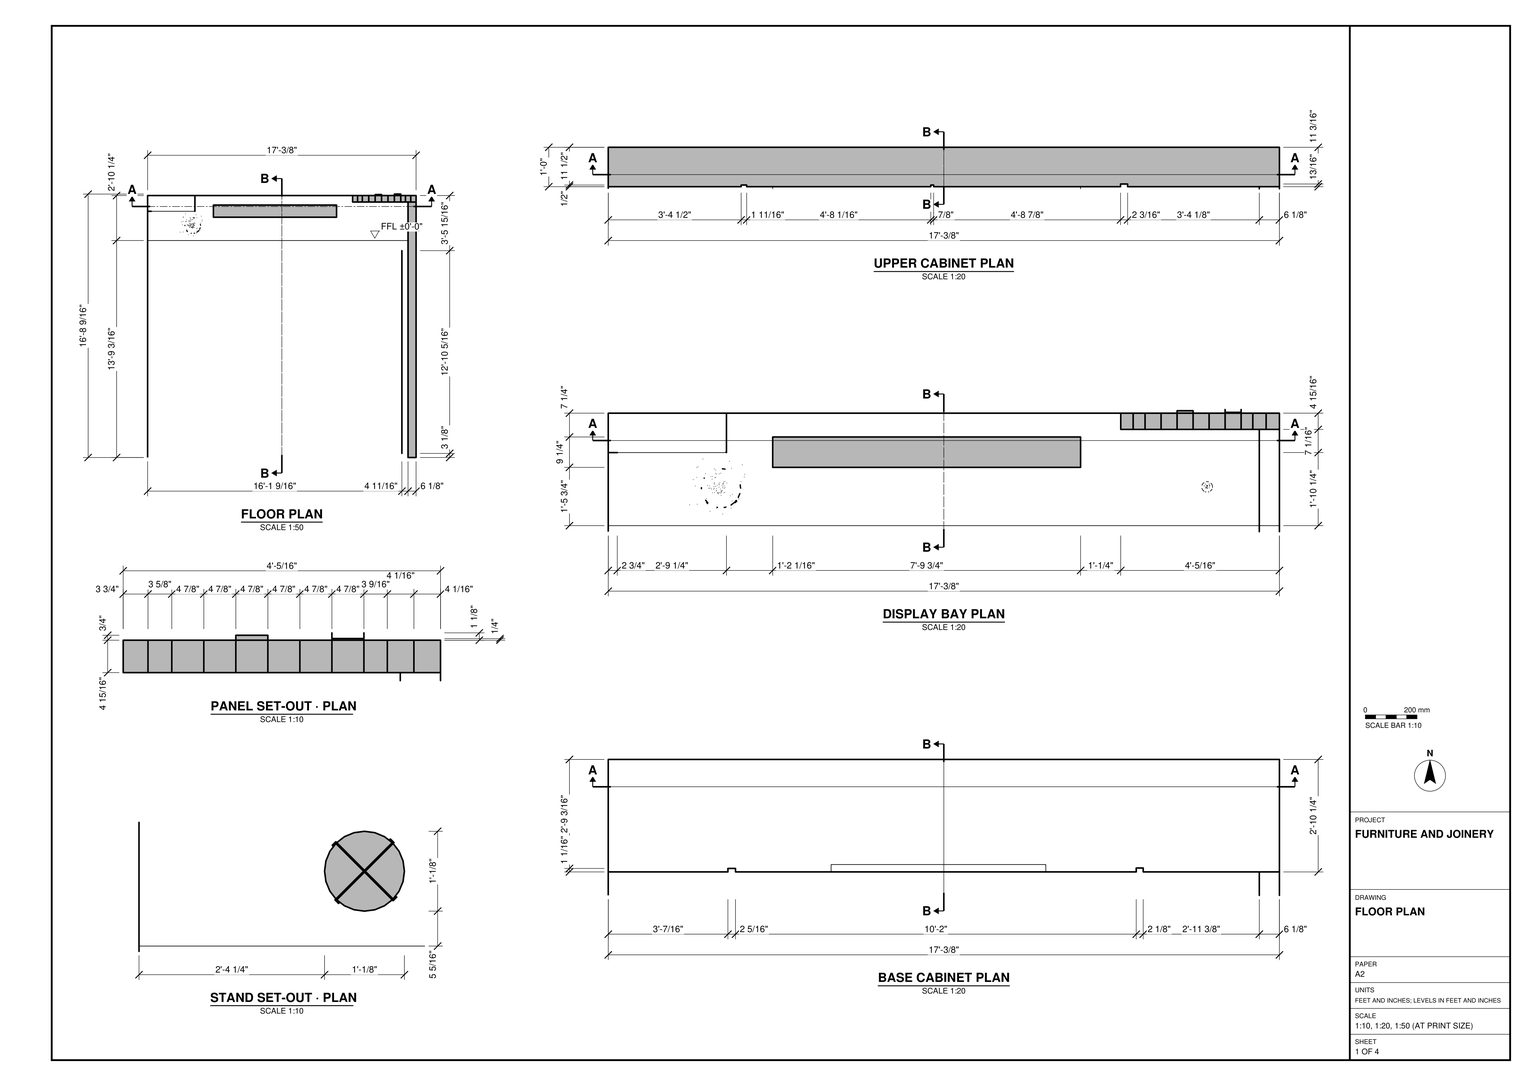
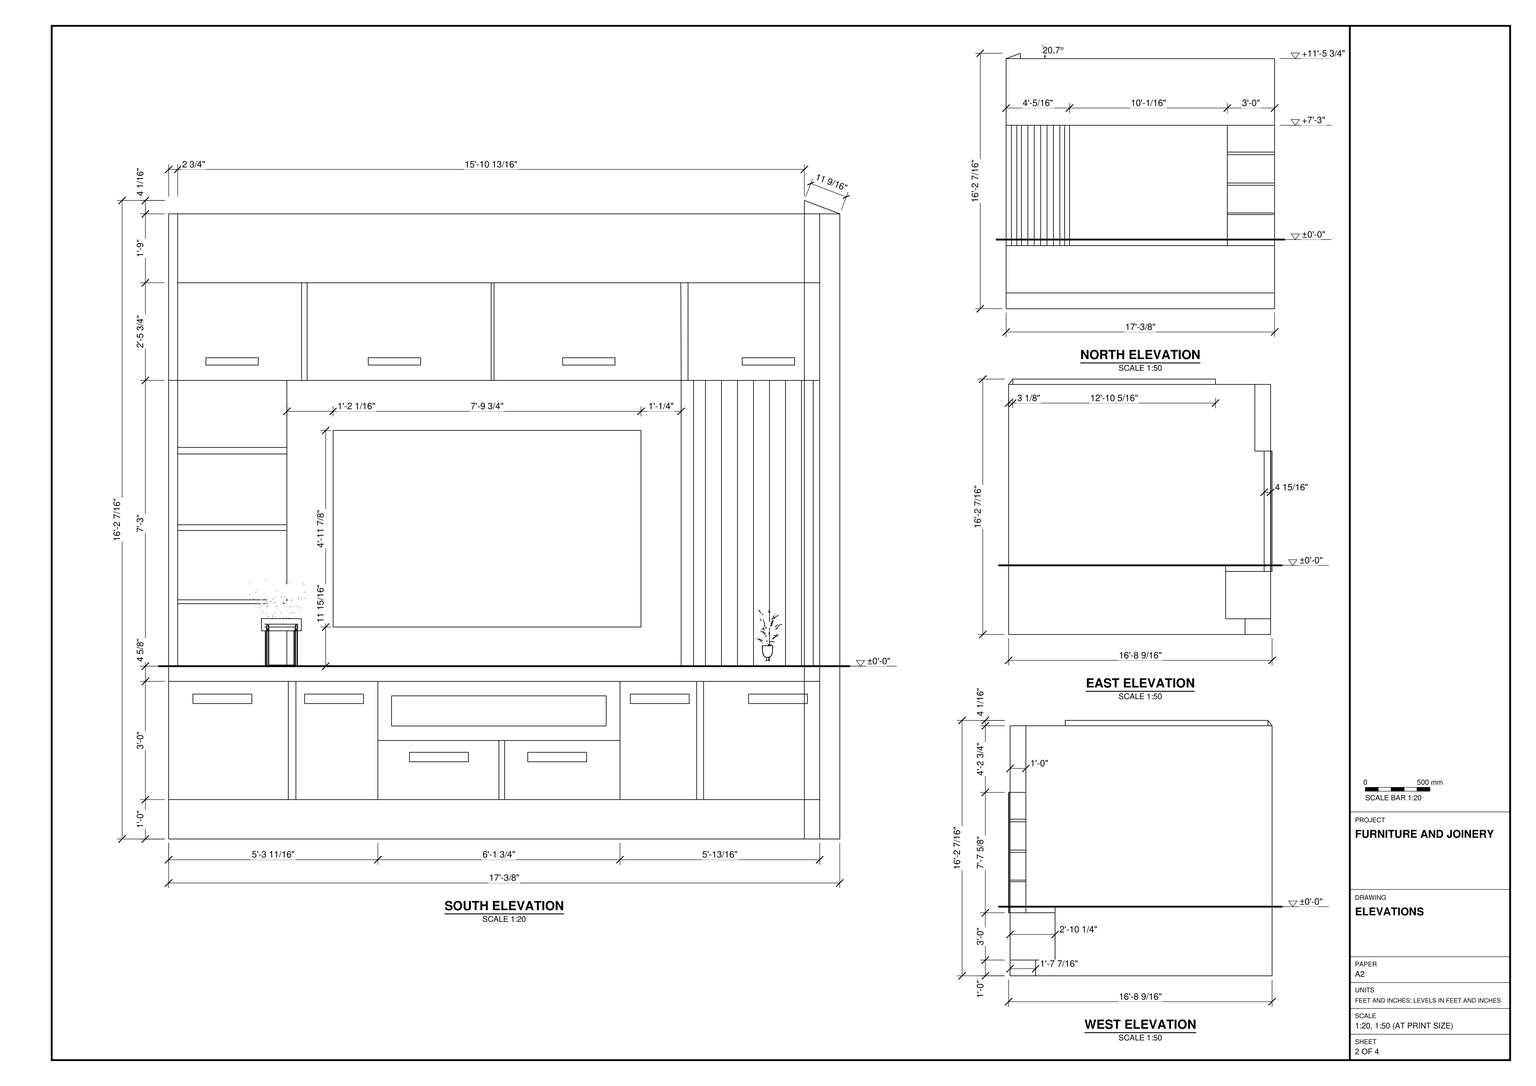
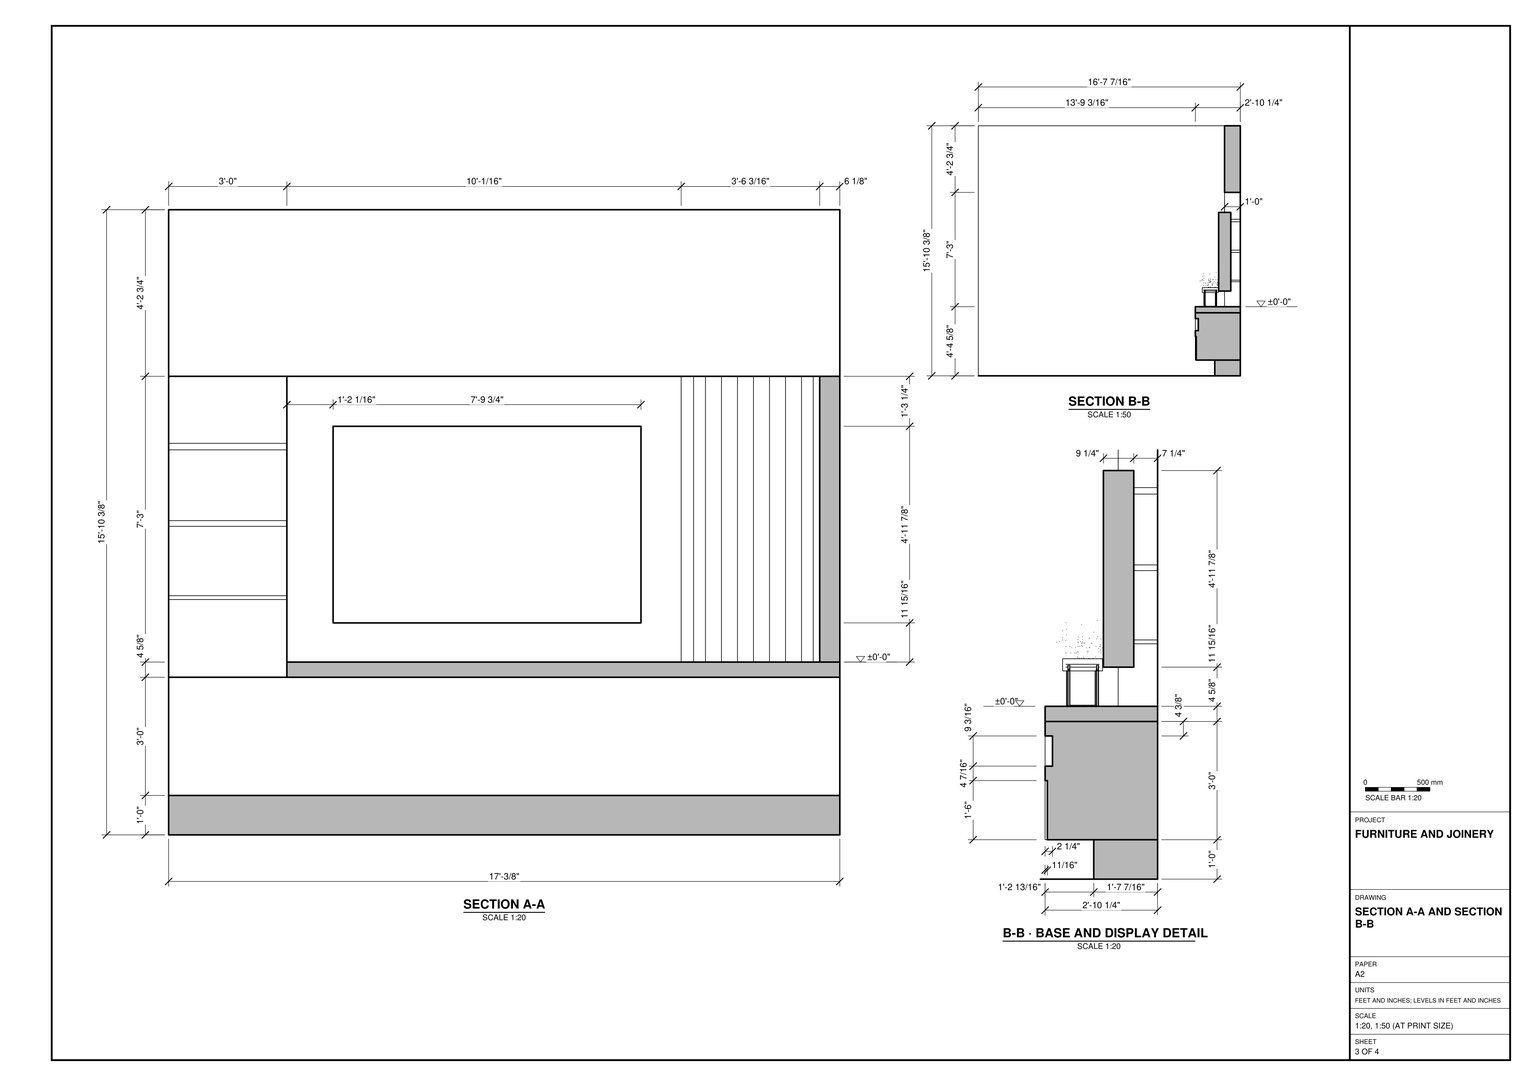
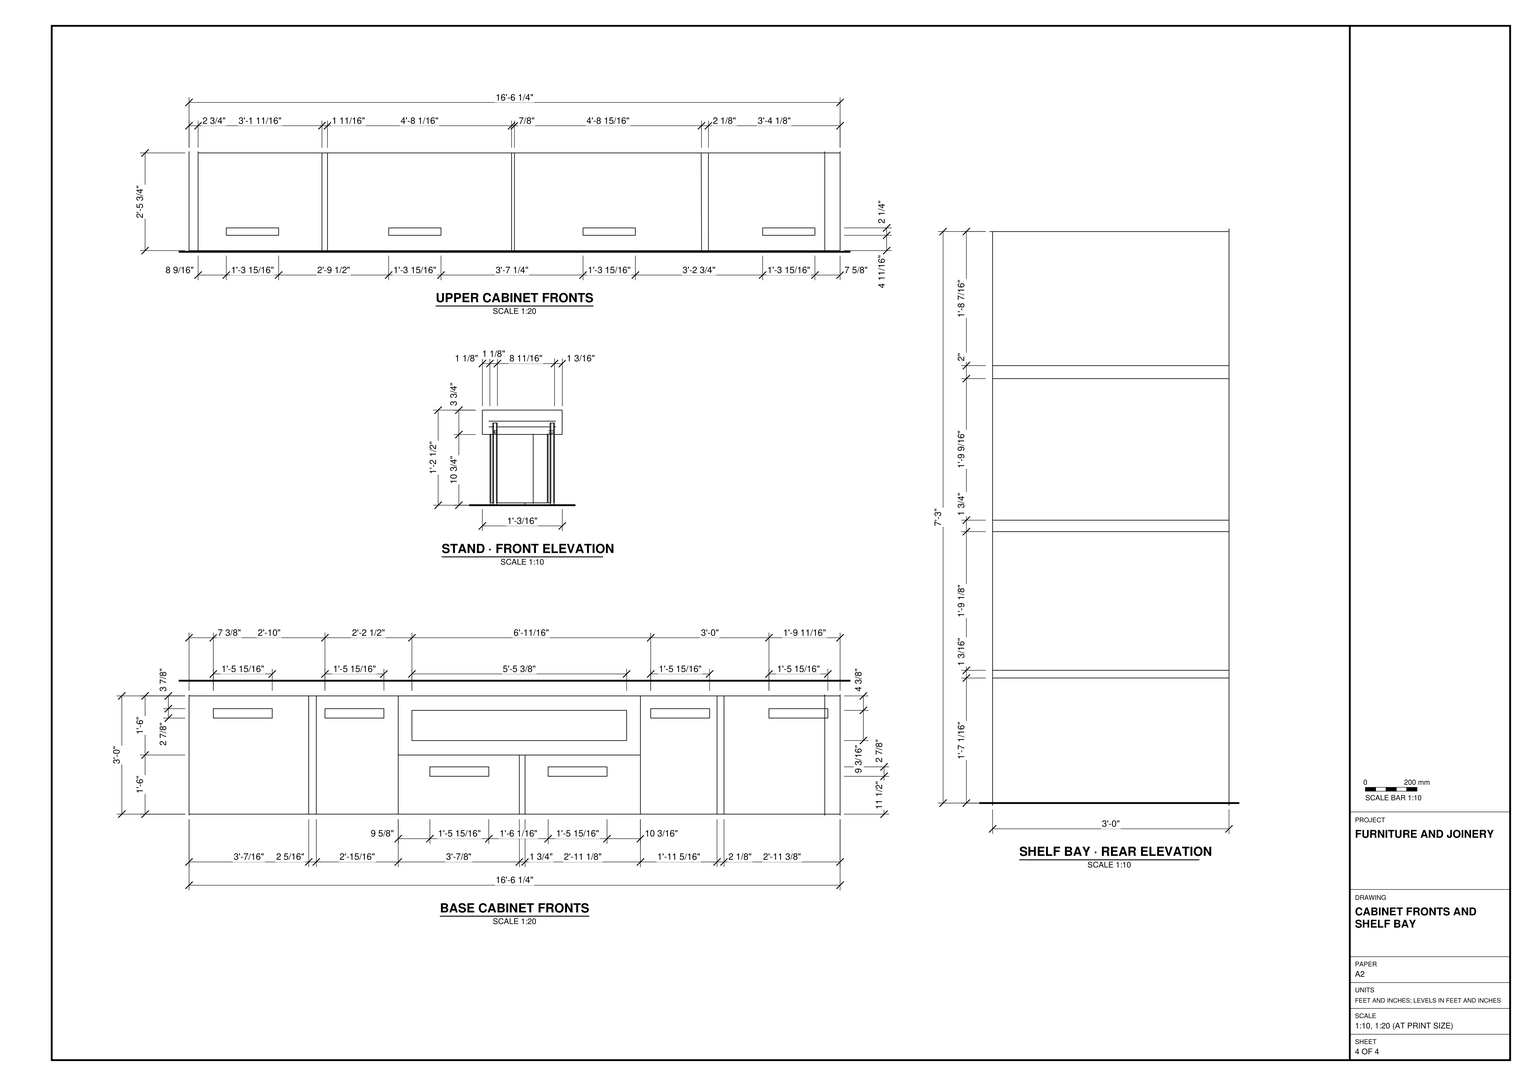
Build the fitted display wall in SketchUp from task_files/diagram_01.pdf. Work in feet and inches. The complete assembly, including the side return, measures 17'-3/8" across the cabinet fronts, 16'-8 9/16" from front to back and 16'-2 7/16" high. Use the marked level of ±0'-0" at the top of the base counter; the base cabinets and their plinth extend below this datum.

Use the south elevation to lay out the cabinet fronts and pulls. Form the recessed plinth, the full-width counter and the central base section with its broad horizontal inset above paired lower fronts. Between the counter and the upper cabinets, place open shelves on the left, a projecting rectangular display panel in the middle and narrow vertical panels on the right. Follow the panel set-out in plan for their widths and offsets. Include the band above the upper cabinet fronts. Use the plans and sections to distinguish the depths of the cabinets, shelves and display panel from the much longer right-hand return, keeping the return thickness as drawn.

Place the small stand and plants where shown; decor and loose items may be any suitable library components. Keep the surrounding elements and each joinery or furniture piece in separate groups or components, and use components for repeated parts. Save one SketchUp model as output_files/display_wall_with_base_and_upper_cabinets.skp.

# SketchUp Ruby script. Lengths in inches.
U = 1.inch
M = Sketchup.active_model
def pt(a) = Geom::Point3d.new(a.map { |v| v * U })
def face(e, loops, mat)
  f = e.add_face(loops[0].map { |a| pt(a) })
  loops[1..].each { |l| e.add_face(l.map { |a| pt(a) }).erase! }
  f.material = f.back_material = mat if mat
  f
end
# faces: each face lists its corners as indices into pts; further lists are holes
def faces(e, pts, list, mat = nil) = list.each { |f| face(e, (f[0].is_a?(Array) ? f : [f]).map { |l| l.map { |i| pts[i] } }, mat) }
# xy, xz, yz: faces in a plane at the given z, y or x. An outline is a flat list of corners, or four numbers for a rectangle; further outlines are holes
def ring(l) = l.size == 4 ? [[l[0], l[1]], [l[2], l[1]], [l[2], l[3]], [l[0], l[3]]] : l.each_slice(2).to_a
def flat(e, list, mat, &to3) = list.each { |f| face(e, (f[0].is_a?(Array) ? f : [f]).map { |l| ring(l).map { |u, v| to3.(u, v) } }, mat) }
def xy(e, z, list, mat = nil) = flat(e, list, mat) { |x, y| [x, y, z] }
def xz(e, y, list, mat = nil) = flat(e, list, mat) { |x, z| [x, y, z] }
def yz(e, x, list, mat = nil) = flat(e, list, mat) { |y, z| [x, y, z] }
def lines(e, pts, list) = list.each { |a, b| e.add_line(pt(pts[a]), pt(pts[b])) }
# prism: a flat outline (further loops are holes) pulled along v
def prism(e, loops, v, mat = nil)
  f = face(e, loops, mat); d = Geom::Vector3d.new(v.map { |x| x * U })
  f.pushpull(f.normal.samedirection?(d) ? d.length : -d.length)
end
def box(e, o, s, mat = nil) = prism(e, [[o, [o[0] + s[0], o[1], o[2]], [o[0] + s[0], o[1] + s[1], o[2]], [o[0], o[1] + s[1], o[2]]]], [0, 0, s[2]], mat)
def at(x, y, z, deg = 0) = Geom::Transformation.translation(pt([x, y, z])) * Geom::Transformation.rotation(ORIGIN, Z_AXIS, deg.degrees)
def axes(o, x, y, z) = Geom::Transformation.new([*x, 0, *y, 0, *z, 0, *pt(o).to_a, 1])
def part(name) = M.definitions.add(name)
# library, detail: a bought-in or finely detailed component or shape, given as its bounding box
def library(name, o, s) = part(name).tap { |d| box(d.entities, o, s) }
def detail(e, o, s) = box(e.add_group.entities, o, s)
def put(e, d, t, mat = nil) = e.add_instance(d, t).tap { |i| i.material = mat if mat }
def group(e, t, mat = nil) = e.add_group.tap { |g| g.transformation = t; g.material = mat if mat }.entities
root = M.entities
M.materials.add("CORTINA").color = [173, 164, 148]
M.materials.add("[Color A01]").color = [255, 204, 204]
M.materials.add("[Color M00]").color = [255, 255, 255]
M.materials.add("[Color M01]").color = [226, 226, 226]
M.materials.add("[Color M08]").color = [30, 30, 30]
M.materials.add("[Fencing Wood Old]").color = [132, 128, 126]
M.materials.add("[Formica Laminate Dark]").color = [50, 53, 60]
M.materials.add("[Formica Speckled Grey]").color = [94, 105, 111]
M.materials.add("[Marble Carrara Gold Floor Tile]").color = [225, 223, 217]
M.materials.add("[Textile_Leaves_Green]").color = [49, 73, 8]
M.materials.add("[Vegetation Bark Ponderosa]").color = [158, 116, 100]
M.materials.add("[Wood Bamboo]").color = [177, 105, 43]
M.materials.add("[Wood Board Cork]").color = [215, 201, 115]
M.materials.add("[Wood Fence]").color = [20, 19, 18]
M.materials.add("[Wood Floor Light]").color = [204, 176, 127]
M.materials.add("[Wood Floor Parquet]").color = [145, 89, 39]
M.materials.add("[Wood Plywood Knots]").color = [137, 122, 41]
c1 = library("Decorative Plant",[-0.35,-0.24,0],[4.14,4.48,6.875])
c2 = part("Cortina")
xz(c2.entities,0,[[0,0,157.48,157.48]],"CORTINA")
c3 = part("curtain")
put(c3.entities,c2,at(0,0,0))
c4 = part("cof")
g1 = group(c4.entities,at(3.92,3.93,-15.01))
xy(g1,0,[[1.97,-0.53,12.72,10.22,22.38,0.56,23.8,1.97,13.05,12.72,22.72,22.38,21.3,23.8,10.55,13.05,0.89,22.72,-0.53,21.3,10.22,10.55,0.56,0.89]],"[Wood Fence]")
xy(g1,0.47,[[1.99,-0.5,0.58,0.91,10.22,10.55,-0.5,21.28,0.91,22.69,10.55,13.05,21.28,23.78,22.69,22.36,13.05,12.72,23.78,1.99,22.36,0.58,12.72,10.22]],"[Wood Fence]")
xy(g1,14.49,[[0.67,0.33,11.64,11.3,22.61,0.33,22.9375,0.67,11.97,11.64,22.9375,22.61,22.61,22.9375,11.64,11.97,0.67,22.9375,0.33,22.61,11.3,11.64,0.33,0.67]],"[Wood Fence]")
xy(g1,14.96,[[0.67,0.33,0.33,0.67,11.3,11.64,0.33,22.61,0.67,22.93,11.64,11.97,22.61,22.9375,22.77,22.77,22.9375,22.61,11.97,11.64,22.93,0.67,22.77,0.5,22.6,0.34,11.64,11.3],[22.6,0.34,22.93,0.67,22.77,0.5],[22.77,0.5,22.93,0.67,24.02,1.75]],"[Wood Fence]")
xy(g1,16.54,[[1.42,-1.08,0,0.33,0.33,0.67,1.75,-0.75],[22.9375,0,22.61,0.33,22.77,0.5,24.02,1.75,24.36,1.42],[-0.75,21.52,-1.08,21.86,0.33,23.27,0.67,22.9375,0.5,22.77],[22.9375,22.61,22.77,22.77,21.52,24.02,21.86,24.36,23.27,22.9375]],"[Wood Fence]")
p = [[12.72,10.22,0],[1.97,-0.53,0],[1.83,-0.67,0.03],[1.69,-0.8,0.11],[1.58,-0.92,0.23],[1.49,-1.01,0.39],
  [1.44,-1.0625,0.58],[1.42,-1.08,0.79],[1.42,-1.08,16.54],[1.75,-0.75,16.54],[1.75,-0.75,14.96],[1.75,-0.75,14.49],
  [1.75,-0.75,0.82],[1.76,-0.74,0.71],[1.78,-0.72,0.63],[1.82,-0.68,0.57],[1.86,-0.64,0.52],[1.92,-0.58,0.49],
  [1.99,-0.5,0.47],[12.72,10.22,0.47],[0.28,0.61,0.11],[0.41,0.75,0.03],[0.56,0.89,0],[22.36,0.58,0.47],
  [22.4375,0.5,0.49],[22.49,0.45,0.52],[22.54,0.4,0.57],[22.57,0.37,0.63],[22.59,0.34,0.71],[22.61,0.33,0.82],
  [22.61,0.33,14.49],[22.6,0.34,14.96],[22.61,0.33,16.54],[22.9375,0,16.54],[22.9375,0,0.79],[22.92,0.02,0.58],
  [22.86,0.07,0.39],[22.78,0.16,0.23],[22.66,0.28,0.11],[22.53,0.41,0.03],[22.38,0.56,0],[10.22,10.55,0.47],
  [0.58,0.91,0.47],[0.5,0.83,0.49],[0.45,0.78,0.52],[0.4,0.74,0.57],[0.37,0.7,0.63],[0.34,0.68,0.71],
  [0.33,0.67,0.82],[0.33,0.67,14.49],[0.33,0.67,14.96],[0.33,0.67,16.54],[0,0.33,16.54],[0,0.33,0.79],
  [0.02,0.35,0.58],[0.07,0.41,0.39],[0.16,0.5,0.23],[10.22,10.55,0],[24.08,1.69,0.11],[23.94,1.83,0.03],
  [23.8,1.97,0],[13.05,12.72,0],[24.19,1.58,0.23],[24.28,1.49,0.39],[24.34,1.44,0.58],[24.36,1.42,0.79],
  [24.36,1.42,16.54],[24.02,1.75,16.54],[24.02,1.75,14.96],[24.02,1.75,14.49],[24.02,1.75,0.82],[24.01,1.76,0.71],
  [23.99,1.78,0.63],[23.95,1.82,0.57],[23.91,1.86,0.52],[23.86,1.92,0.49],[23.78,1.99,0.47],[13.05,12.72,0.47],
  [-0.53,21.3,0],[-0.67,21.44,0.03],[-0.8,21.58,0.11],[-0.92,21.69,0.23],[-1.01,21.78,0.39],[-1.0625,21.84,0.58],
  [-1.08,21.86,0.79],[-1.08,21.86,16.54],[-0.75,21.52,16.54],[-0.75,21.52,14.96],[-0.75,21.52,14.49],[-0.75,21.52,0.82],
  [-0.74,21.51,0.71],[-0.72,21.49,0.63],[-0.68,21.46,0.57],[-0.64,21.41,0.52],[-0.58,21.36,0.49],[-0.5,21.28,0.47],
  [22.69,22.36,0.47],[22.77,22.4375,0.49],[22.83,22.49,0.52],[22.87,22.54,0.57],[22.91,22.57,0.63],[22.93,22.59,0.71],
  [22.9375,22.61,0.82],[22.9375,22.61,14.49],[22.9375,22.61,14.96],[22.9375,22.61,16.54],[23.27,22.9375,16.54],[23.27,22.9375,0.79],
  [23.25,22.92,0.58],[23.2,22.86,0.39],[23.11,22.78,0.23],[22.99,22.66,0.11],[22.86,22.53,0.03],[22.72,22.38,0],
  [10.55,13.05,0.47],[0.91,22.69,0.47],[0.83,22.77,0.49],[0.78,22.83,0.52],[0.74,22.87,0.57],[0.7,22.91,0.63],
  [0.68,22.93,0.71],[0.67,22.9375,0.82],[0.67,22.9375,14.49],[0.67,22.93,14.96],[0.67,22.9375,16.54],[0.33,23.27,16.54],
  [0.33,23.27,0.79],[0.35,23.25,0.58],[0.41,23.2,0.39],[0.5,23.11,0.23],[0.61,22.99,0.11],[0.75,22.86,0.03],
  [0.89,22.72,0],[10.55,13.05,0],[21.3,23.8,0],[21.44,23.94,0.03],[21.58,24.08,0.11],[21.69,24.19,0.23],
  [21.78,24.28,0.39],[21.84,24.34,0.58],[21.86,24.36,0.79],[21.86,24.36,16.54],[21.52,24.02,16.54],[21.52,24.02,14.96],
  [21.52,24.02,14.49],[21.52,24.02,0.82],[21.51,24.01,0.71],[21.49,23.99,0.63],[21.46,23.95,0.57],[21.41,23.91,0.52],
  [21.36,23.86,0.49],[21.28,23.78,0.47],[0.67,0.33,14.49],[22.9375,0.67,14.49],[0.33,22.61,14.49],[22.61,22.9375,14.49],
  [0.67,0.33,14.96],[0.5,0.5,14.96],[11.64,11.3,14.49],[11.64,11.3,14.96],[22.93,0.67,14.96],[11.3,11.64,14.96],
  [11.3,11.64,14.49],[11.97,11.64,14.49],[11.97,11.64,14.96],[0.33,22.61,14.96],[11.64,11.97,14.96],[11.64,11.97,14.49],
  [22.61,22.9375,14.96],[22.77,22.77,14.96],[0.5,0.5,16.54],[22.77,0.5,14.96],[22.77,0.5,16.54],[0.5,22.77,16.54],
  [0.5,22.77,14.96],[22.77,22.77,16.54]]
faces(g1,p,[[0,1,2,3,4,5,6,7,8,9,10,11,12,13,14,15,16,17,18,19],[20,3,2,21],[21,2,1,22],[19,23,24,25,26,27,28,29,30,31,32,33,34,35,36,37,38,39,40,0],[41,42,43,44,45,46,47,48,49,50,51,52,53,54,55,56,20,21,22,57],[39,38,58,59],[40,39,59,60],[61,60,59,58,62,63,64,65,66,67,68,69,70,71,72,73,74,75,76,77],
  [57,78,79,80,81,82,83,84,85,86,87,88,89,90,91,92,93,94,95,41],[77,96,97,98,99,100,101,102,103,104,105,106,107,108,109,110,111,112,113,61],[114,115,116,117,118,119,120,121,122,123,124,125,126,127,128,129,130,131,132,133],[133,134,135,136,137,138,139,140,141,142,143,144,145,146,147,148,149,150,151,114],[131,79,78,132],[130,80,79,131],[113,112,135,134],[112,111,136,135],
  [56,4,3,20],[38,37,62,58],[129,81,80,130],[111,110,137,136],[55,5,4,56],[37,36,63,62],[128,82,81,129],[110,109,138,137],
  [54,6,5,55],[36,35,64,63],[127,83,82,128],[109,108,139,138],[44,16,15,45],[43,17,16,44],[42,18,17,43],[25,24,75,74],
  [26,25,74,73],[24,23,76,75],[115,95,94,116],[117,93,92,118],[116,94,93,117],[97,96,151,150],[98,97,150,149],[99,98,149,148],
  [53,7,6,54],[46,14,13,47],[45,15,14,46],[35,34,65,64],[28,27,72,71],[27,26,73,72],[119,91,90,120],[118,92,91,119],
  [126,84,83,127],[100,99,148,147],[101,100,147,146],[108,107,140,139],[47,13,12,48],[29,28,71,70],[120,90,89,121],[102,101,146,145],
  [52,8,7,53],[49,48,12,11,152],[34,33,66,65],[30,29,70,69,153],[122,121,89,88,154],[125,85,84,126],[103,102,145,144,155],[107,106,141,140],
  [156,152,11,10],[156,152,49,50,157],[158,152,156,159],[159,31,30,158],[30,31,153],[160,153,31],[161,50,49,162],[163,153,160,164],
  [153,69,160],[68,160,69],[162,154,165,161],[164,104,103,163],[166,123,122,167],[167,155,168,166],[165,154,88,87],[122,123,154],
  [165,154,123],[103,104,169,168,155],[168,155,144,143],[9,170,157,156,10],[171,172,31],[32,31,172],[50,157,170,51],[172,171,68],
  [67,172,68],[86,173,174,165,87],[104,169,175,105],[174,173,123],[124,123,173],[142,175,169,168,143]],"[Wood Fence]")
c5 = part("Component")
g2 = group(c5.entities,at(0,0,0),"[Vegetation Bark Ponderosa]")
put(g2,c4,axes([-4.91,2.93,5.08],[0.07854,0,0],[0,0.07854,0],[0,0,0.34302]),"[Fencing Wood Old]")
g3 = group(g2,at(-4.92,2.91,4.8125),"[Vegetation Bark Ponderosa]")
xy(g3,0.52,[[1.24,0.04,1.55,0.08,1.83,0.2,2.08,0.39,2.27,0.64,2.39,0.93,2.43,1.24,2.39,1.55,2.27,1.83,2.08,2.08,1.83,2.27,1.55,2.39,1.24,2.43,0.93,2.39,0.64,2.27,0.39,2.08,0.2,1.83,0.08,1.55,0.04,1.24,0.08,0.93,0.2,0.64,0.39,0.39,0.64,0.2,0.93,0.08]],"[Vegetation Bark Ponderosa]")
xy(g3,0.92,[[1.24,0.04,1.55,0.08,1.83,0.2,2.08,0.39,2.27,0.64,2.39,0.93,2.43,1.24,2.39,1.55,2.27,1.83,2.08,2.08,1.83,2.27,1.55,2.39,1.24,2.43,0.93,2.39,0.64,2.27,0.39,2.08,0.2,1.83,0.08,1.55,0.04,1.24,0.08,0.93,0.2,0.64,0.39,0.39,0.64,0.2,0.93,0.08]],"[Vegetation Bark Ponderosa]")
xy(g3,1.68,[[[1.24,0,1.56,0.04,1.86,0.17,2.11,0.36,2.31,0.62,2.43,0.92,2.47,1.24,2.43,1.56,2.31,1.86,2.11,2.11,1.86,2.31,1.56,2.43,1.24,2.47,0.92,2.43,0.62,2.31,0.36,2.11,0.17,1.86,0.04,1.56,0,1.24,0.04,0.92,0.17,0.62,0.36,0.36,0.62,0.17,0.92,0.04],[1.24,0.04,0.93,0.08,0.64,0.2,0.39,0.39,0.2,0.64,0.08,0.93,0.04,1.24,0.08,1.55,0.2,1.83,0.39,2.08,0.64,2.27,0.93,2.39,1.24,2.43,1.55,2.39,1.83,2.27,2.08,2.08,2.27,1.83,2.39,1.55,2.43,1.24,2.39,0.93,2.27,0.64,2.08,0.39,1.83,0.2,1.55,0.08]]],"[Color M00]")
p = [[0.62,0.17,0],[0.92,0.04,0],[0.92,0.04,1.68],[0.62,0.17,1.68],[1.24,0,0],[1.24,0,1.68],
  [1.56,0.04,0],[1.56,0.04,1.68],[1.86,0.17,0],[1.86,0.17,1.68],[0.36,0.36,0],[0.36,0.36,1.68],
  [2.11,0.36,0],[2.11,0.36,1.68],[0.17,0.62,0],[0.17,0.62,1.68],[2.31,0.62,0],[2.31,0.62,1.68],
  [0.04,0.92,0],[0.04,0.92,1.68],[2.43,0.92,0],[2.43,0.92,1.68],[0,1.24,0],[0,1.24,1.68],
  [2.47,1.24,0],[2.47,1.24,1.68],[0.04,1.56,0],[0.04,1.56,1.68],[2.43,1.56,0],[2.43,1.56,1.68],
  [0.17,1.86,0],[0.17,1.86,1.68],[2.31,1.86,0],[2.31,1.86,1.68],[0.36,2.11,0],[0.36,2.11,1.68],
  [2.11,2.11,0],[2.11,2.11,1.68],[0.62,2.31,0],[0.62,2.31,1.68],[1.86,2.31,0],[1.86,2.31,1.68],
  [0.92,2.43,0],[0.92,2.43,1.68],[1.56,2.43,0],[1.56,2.43,1.68],[1.24,2.47,0],[1.24,2.47,1.68],
  [1.24,0.04,0.52],[0.93,0.08,0.52],[0.93,0.08,0.92],[1.24,0.04,0.92],[1.55,0.08,0.52],[1.55,0.08,0.92],
  [0.64,0.2,0.52],[0.64,0.2,0.92],[1.83,0.2,0.52],[1.83,0.2,0.92],[0.39,0.39,0.52],[0.39,0.39,0.92],
  [2.08,0.39,0.52],[2.08,0.39,0.92],[0.2,0.64,0.52],[0.2,0.64,0.92],[2.27,0.64,0.52],[2.27,0.64,0.92],
  [0.08,0.93,0.52],[0.08,0.93,0.92],[2.39,0.93,0.52],[2.39,0.93,0.92],[0.04,1.24,0.52],[0.04,1.24,0.92],
  [2.43,1.24,0.52],[2.43,1.24,0.92],[0.08,1.55,0.52],[0.08,1.55,0.92],[2.39,1.55,0.52],[2.39,1.55,0.92],
  [0.2,1.83,0.52],[0.2,1.83,0.92],[2.27,1.83,0.52],[2.27,1.83,0.92],[0.39,2.08,0.52],[0.39,2.08,0.92],
  [2.08,2.08,0.52],[2.08,2.08,0.92],[0.64,2.27,0.52],[0.64,2.27,0.92],[1.83,2.27,0.52],[1.83,2.27,0.92],
  [0.93,2.39,0.52],[0.93,2.39,0.92],[1.55,2.39,0.52],[1.55,2.39,0.92],[1.24,2.43,0.52],[1.24,2.43,0.92],
  [1.24,0.04,1.68],[0.93,0.08,1.68],[1.55,0.08,1.68],[0.64,0.2,1.68],[1.83,0.2,1.68],[0.39,0.39,1.68],
  [2.08,0.39,1.68],[0.2,0.64,1.68],[2.27,0.64,1.68],[0.08,0.93,1.68],[2.39,0.93,1.68],[0.04,1.24,1.68],
  [2.43,1.24,1.68],[0.08,1.55,1.68],[2.39,1.55,1.68],[0.2,1.83,1.68],[2.27,1.83,1.68],[0.39,2.08,1.68],
  [2.08,2.08,1.68],[0.64,2.27,1.68],[1.83,2.27,1.68],[0.93,2.39,1.68],[1.55,2.39,1.68],[1.24,2.43,1.68]]
faces(g3,p,[[0,1,2,3],[1,4,5,2],[4,6,7,5],[6,8,9,7],[10,0,3,11],[8,12,13,9],[14,10,11,15],[12,16,17,13],
  [18,14,15,19],[16,20,21,17],[22,18,19,23],[20,24,25,21],[26,22,23,27],[24,28,29,25],[30,26,27,31],[28,32,33,29],
  [34,30,31,35],[32,36,37,33],[38,34,35,39],[36,40,41,37],[42,38,39,43],[40,44,45,41],[46,42,43,47],[44,46,47,45],
  [96,51,50,97],[98,53,51,96],[97,50,55,99],[100,57,53,98],[99,55,59,101],[102,61,57,100],[101,59,63,103],[104,65,61,102],
  [103,63,67,105],[106,69,65,104],[105,67,71,107],[108,73,69,106],[107,71,75,109],[110,77,73,108],[109,75,79,111],[112,81,77,110],
  [111,79,83,113],[114,85,81,112],[113,83,87,115],[116,89,85,114],[115,87,91,117],[118,93,89,116],[117,91,95,119],[119,95,93,118]],"[Color M00]")
faces(g3,p,[[48,49,50,51],[52,48,51,53],[49,54,55,50],[56,52,53,57],[54,58,59,55],[60,56,57,61],[58,62,63,59],[64,60,61,65],
  [62,66,67,63],[68,64,65,69],[66,70,71,67],[72,68,69,73],[70,74,75,71],[76,72,73,77],[74,78,79,75],[80,76,77,81],
  [78,82,83,79],[84,80,81,85],[82,86,87,83],[88,84,85,89],[86,90,91,87],[92,88,89,93],[90,94,95,91],[94,92,93,95]],"[Vegetation Bark Ponderosa]")
c6 = part("Plant leaf")
p = [[4.001,2.211,9.034],[3.964,2.195,9.038],[2.645,1.619,9.164],[2.684,1.471,8.407],[2.728,1.324,7.649],[2.778,1.18,6.891],
  [2.834,1.039,6.133],[2.895,0.9,5.374],[2.962,0.764,4.614],[3.035,0.631,3.855],[3.114,0.499,3.095],[3.198,0.371,2.334],
  [3.288,0.245,1.574],[3.383,0.121,0.8125],[3.485,0,0.051],[3.964,0.209,0.004],[4.001,0.225,0],[3.926,2.211,9.034],
  [3.926,0.225,0],[4.443,0,0.051],[4.544,0.121,0.8125],[4.64,0.245,1.574],[4.73,0.371,2.334],[4.814,0.499,3.095],
  [4.892,0.631,3.855],[4.965,0.764,4.614],[5.032,0.9,5.374],[5.094,1.039,6.133],[5.15,1.18,6.891],[5.2,1.324,7.649],
  [5.244,1.471,8.407],[5.283,1.619,9.164],[4.001,5.314,17.748],[3.964,5.299,17.754],[2.264,4.583,18.009],[2.638,1.639,9.243],
  [3.964,2.196,9.04],[2.638,1.638,9.241],[5.29,1.639,9.243],[5.29,1.638,9.241],[3.926,5.314,17.748],[5.664,4.583,18.009],
  [4.001,9.442,26.026],[3.964,9.427,26.034],[2.001,8.641,26.425],[1.959,8.281,25.744],[1.929,7.925,25.061],[1.91,7.574,24.375],
  [1.903,7.227,23.686],[1.907,6.884,22.996],[1.922,6.547,22.303],[1.949,6.213,21.608],[1.987,5.885,20.911],[2.036,5.561,20.211],
  [2.097,5.242,19.51],[2.17,4.928,18.807],[2.253,4.618,18.102],[3.964,5.299,17.756],[5.674,4.618,18.102],[3.926,9.442,26.026],
  [5.758,4.928,18.807],[5.83,5.242,19.51],[5.891,5.561,20.211],[5.941,5.885,20.911],[5.979,6.213,21.608],[6.006,6.547,22.303],
  [6.021,6.884,22.996],[6.025,7.227,23.686],[6.018,7.574,24.375],[5.999,7.925,25.061],[5.969,8.281,25.744],[5.927,8.641,26.425],
  [3.964,9.428,26.035],[2.001,8.688,26.507],[5.927,8.688,26.507],[4.001,14.357,33.862],[3.964,14.343,33.871],[2.87,13.929,34.131],
  [2.735,13.47,33.513],[2.611,13.015,32.891],[2.499,12.564,32.267],[2.398,12.117,31.639],[2.309,11.674,31.008],[2.23,11.235,30.374],
  [2.164,10.8,29.737],[2.108,10.369,29.097],[2.064,9.942,28.454],[2.032,9.52,27.808],[2.011,9.102,27.159],[3.926,14.357,33.862],
  [5.917,9.102,27.159],[5.896,9.52,27.808],[5.863,9.942,28.454],[5.819,10.369,29.097],[5.764,10.8,29.737],[5.697,11.235,30.374],
  [5.619,11.674,31.008],[5.53,12.117,31.639],[5.429,12.564,32.267],[5.316,13.015,32.891],[5.193,13.47,33.513],[5.058,13.929,34.131],
  [3.964,14.344,33.873],[2.869,13.975,34.194],[5.058,13.975,34.194],[4.001,20.377,40.886],[3.97,19.863,40.308],[3.964,19.793,40.23],
  [3.927,19.346,39.734],[3.872,18.825,39.163],[3.806,18.3,38.596],[3.729,17.771,38.033],[3.64,17.24,37.473],[3.54,16.704,36.917],
  [3.428,16.165,36.365],[3.306,15.623,35.817],[3.171,15.077,35.272],[3.026,14.528,34.731],[3.926,20.377,40.886],[4.902,14.528,34.731],
  [4.756,15.077,35.272],[4.622,15.623,35.817],[4.499,16.165,36.365],[4.388,16.704,36.917],[4.288,17.24,37.473],[4.199,17.771,38.033],
  [4.122,18.3,38.596],[4.056,18.825,39.163],[4.001,19.346,39.734],[3.958,19.863,40.308]]
faces(c6.entities,p,[[0,1,2,3,4,5,6,7,8,9,10,11,12,13,14,15,16],[1,17,18,15,19,20,21,22,23,24,25,26,27,28,29,30,31],[32,33,34,35,36,0],[36,35,37,2,1,0],[38,36,17,1,31,39],[33,40,17,36,38,41],[42,43,44,45,46,47,48,49,50,51,52,53,54,55,56,57,32],[57,56,34,33,32],
  [58,57,40,33,41],[43,59,40,57,58,60,61,62,63,64,65,66,67,68,69,70,71],[72,73,44,43,42],[74,72,59,43,71],[75,76,77,78,79,80,81,82,83,84,85,86,87,88,73,72,42],[76,89,59,72,74,90,91,92,93,94,95,96,97,98,99,100,101],[102,103,77,76,75],[104,102,89,76,101],
  [75,105,106,107,108,109,110,111,112,113,114,115,116,117,103,102],[118,89,102,104,119,120,121,122,123,124,125,126,127,128,107,129]],"[Textile_Leaves_Green]")
xy(root,0,[[198.25,0,204.375,180],[0,180,204.375,199.4375]])
xy(root,0,[[0,0,198.25,180]],"[Marble Carrara Gold Floor Tile]")
xy(root,12,[[0,165.1875,0,180,198.25,180,198.25,165.1875,162.9,165.1875,162.9,166.375,160.78,166.375,160.78,165.1875,102.32,165.1875,102.32,165.875,100.57,165.875,100.57,165.1875,38.75,165.1875,38.75,166.25,36.4375,166.25,36.4375,165.1875],[198.25,165.1875,204.375,180],[0,180,204.375,199.4375]])
xy(root,30,[[100.57,165.1875,102.32,165.875]])
xy(root,34.41,[[67.87,165.1875,133.24,167.4375]],"[Wood Board Cork]")
xy(root,43.6,[[67.87,165.1875,133.24,167.4375]])
xy(root,48,[[0,165.1875,0,187.4375,36,187.4375,36,199.4375,156.0625,199.4375,156.0625,194.5,204.375,194.5,204.375,165.1875,162.9,165.1875,162.9,166.375,160.78,166.375,160.78,165.1875,38.75,165.1875,38.75,166.25,36.4375,166.25,36.4375,165.1875],[36.4375,165.1875,38.75,166.25],[160.78,165.1875,162.9,166.375],[156.0625,194.5,159.84,199.4375],[159.84,194.5,163.46,199.4375],
  [163.46,194.5,168.34,199.4375],[168.34,194.5,173.21,199.4375],[173.21,194.5,178.09,199.4375],[178.09,194.5,182.96,199.4375],[182.96,194.5,187.84,199.4375],
  [187.84,194.5,192.71,199.4375],[192.71,194.5,196.28,199.4375],[196.28,194.5,200.33,199.4375],[200.33,194.5,204.375,199.4375],[173.21,199.4375,178.09,200.1875],
  [187.84,199.4375,192.71,199.6875],[187.84,199.6875,192.71,200.5625]])
xy(root,48,[[0,187.4375,36,199.4375]],"[Wood Bamboo]")
xy(root,52.625,[[198.25,165.1875,204.375,194.5]])
xy(root,52.625,[[0,165.1875,198.25,165.1875,198.25,194.5,156.0625,194.5,156.0625,199.4375,36,199.4375,36,187.4375,0,187.4375]],"[Wood Floor Light]")
xy(root,139.64,[[158.15,187.4375,158.15,188.25,156.0625,188.25,156.0625,194.5,198.25,194.5,198.25,187.4375],[198.25,187.4375,204.375,194.5],[156.0625,194.5,159.84,199.4375],[159.84,194.5,163.46,199.4375],[163.46,194.5,168.34,199.4375],
  [168.34,194.5,173.21,199.4375],[173.21,194.5,178.09,199.4375],[178.09,194.5,182.96,199.4375],[182.96,194.5,187.84,199.4375],[187.84,194.5,192.71,199.4375],
  [192.71,194.5,196.28,199.4375],[196.28,194.5,200.33,199.4375],[200.33,194.5,204.375,199.4375],[173.21,199.4375,178.09,200.1875],[187.84,199.4375,192.71,199.6875],
  [187.84,199.6875,192.71,200.5625]])
xy(root,139.64,[[0,187.4375,36,199.4375],[36,187.4375,36,199.4375,156.0625,199.4375,156.0625,187.4375,99.09,187.4375,99.09,187.9375,98.21,187.9375,98.21,187.4375,42.16,187.4375,42.16,187.9375,40.47,187.9375,40.47,187.4375]],"[Wood Bamboo]")
xy(root,169.39,[[40.47,187.4375,42.16,187.9375],[98.21,187.4375,99.09,187.9375],[155.96,187.4375,156.39,188.25],[156.39,187.4375,158.15,188.25]])
xy(root,190.375,[[198.25,0,204.375,187.4375]],"[Color A01]")
xy(root,190.375,[[0,187.4375,204.375,199.4375]],"[Wood Floor Parquet]")
xz(root,0,[[198.25,0,204.375,190.375]],"[Color A01]")
xz(root,165.1875,[[198.25,12,204.375,48],[198.25,48,204.375,52.625]])
xz(root,165.1875,[[[0,12,36.4375,48],[7.39,41.25,25.33,44.125]],[[38.75,12,63.69,48],[41.39,41.25,59.33,44.125]],[[63.69,12,100.57,30],[73.34,23.52,91.28,26.39]],[[102.32,12,137.45,30],[109.34,23.52,127.28,26.39]],[[137.45,12,160.78,48],[140.58,41.25,158.52,44.125]],
  [[162.9,12,198.25,48],[176.58,41.25,194.52,44.125]],[[63.69,30,137.45,48],[67.87,34.41,133.24,43.6]],[0,48,198.25,52.625]],"[Wood Floor Light]")
xz(root,165.1875,[[73.34,23.52,91.28,26.39],[109.34,23.52,127.28,26.39],[7.39,41.25,25.33,44.125],[41.39,41.25,59.33,44.125],[140.58,41.25,158.52,44.125],
  [176.58,41.25,194.52,44.125]],"[Wood Plywood Knots]")
xz(root,165.875,[[100.57,12,102.32,30]],"[Formica Speckled Grey]")
xz(root,166.25,[[36.4375,12,38.75,48]],"[Formica Speckled Grey]")
xz(root,166.375,[[160.78,12,162.9,48]],"[Formica Speckled Grey]")
xz(root,167.4375,[[67.87,34.41,133.24,43.6]],"[Wood Board Cork]")
xz(root,180,[[198.25,0,204.375,12]])
xz(root,180,[[0,0,198.25,12]],"[Wood Bamboo]")
xz(root,187.4375,[[0,48,2.75,52.625],[2.75,48,36,52.625],[198.25,139.64,204.375,169.39],[198.25,169.39,204.375,190.375]])
xz(root,187.4375,[[11.35,144.31,27.28,146.56],[60.78,144.31,76.72,146.56],[119.97,144.31,135.91,146.56],[174.66,144.31,190.6,146.56]],"[Formica Laminate Dark]")
xz(root,187.4375,[[0,52.625,2.75,139.64],[2.75,71.67,36,72.84],[2.75,93.96,36,95.7],[2.75,117.25,36,119.23],[0,139.64,2.75,190.375]],"[Wood Bamboo]")
xz(root,187.4375,[[[2.75,139.64,40.47,169.39],[11.35,144.31,27.28,146.56]],[[42.16,139.64,98.21,169.39],[60.78,144.31,76.72,146.56]],[[99.09,139.64,156.0625,139.64,155.96,169.39,99.09,169.39],[119.97,144.31,135.91,146.56]],[[158.15,139.64,198.25,169.39],[174.66,144.31,190.6,146.56]],[2.75,169.39,198.25,190.375]],"[Wood Floor Parquet]")
xz(root,187.9375,[[40.47,139.64,42.16,169.39],[98.21,139.64,99.09,169.39]],"[Formica Laminate Dark]")
xz(root,188.25,[[156.0625,139.64,158.15,139.64,158.15,169.39,155.96,169.39]],"[Formica Laminate Dark]")
xz(root,194.5,[[156.0625,48,159.84,52.625],[159.84,48,163.46,52.625],[163.46,48,168.34,52.625],[168.34,48,173.21,52.625],[173.21,48,178.09,52.625],
  [178.09,48,182.96,52.625],[182.96,48,187.84,52.625],[187.84,48,192.71,52.625],[192.71,48,196.28,52.625],[196.28,48,200.33,52.625],
  [200.33,48,204.375,52.625]])
xz(root,194.5,[[156.0625,52.625,159.84,139.64],[159.84,52.625,163.46,139.64],[163.46,52.625,168.34,139.64],[168.34,52.625,173.21,139.64],[173.21,52.625,178.09,139.64],
  [178.09,52.625,182.96,139.64],[182.96,52.625,187.84,139.64],[187.84,52.625,192.71,139.64],[192.71,52.625,196.28,139.64],[196.28,52.625,198.25,139.64],
  [198.25,52.625,200.33,139.64],[200.33,52.625,204.375,139.64]],"[Wood Floor Parquet]")
xz(root,199.4375,[[0,0,204.375,12],[0,12,204.375,48],[36,48,156.0625,52.625],[156.0625,48,159.84,139.64],[159.84,48,163.46,139.64],
  [163.46,48,168.34,139.64],[168.34,48,173.21,139.64],[173.21,48,178.09,139.64],[178.09,48,182.96,139.64],[182.96,48,187.84,139.64],
  [187.84,48,192.71,139.64],[192.71,48,196.28,139.64],[196.28,48,200.33,139.64],[200.33,48,204.375,139.64],[36,52.625,156.0625,139.64],
  [0,139.64,204.375,190.375]])
xz(root,199.4375,[[0,48,36,71.67],[0,72.84,36,93.96],[0,95.7,36,117.25],[0,119.23,36,139.64]],"[Formica Laminate Dark]")
xz(root,199.4375,[[0,71.67,36,72.84],[0,93.96,36,95.7],[0,117.25,36,119.23]],"[Wood Bamboo]")
xz(root,199.6875,[[187.84,48,192.71,139.64]])
xz(root,200.1875,[[173.21,48,178.09,139.64]])
xz(root,200.5625,[[187.84,48,192.71,139.64]])
yz(root,0,[[0,0,0,190.375,187.4375,190.375,187.4375,52.625,165.1875,52.625,165.1875,12,180,12,180,0],[180,0,199.4375,12],[165.1875,12,199.4375,48],[165.1875,48,187.4375,52.625],[187.4375,48,199.4375,71.67],
  [187.4375,72.84,199.4375,93.96],[187.4375,95.7,199.4375,117.25],[187.4375,119.23,199.4375,139.64],[187.4375,139.64,199.4375,190.375]],"[Color A01]")
yz(root,0,[[187.4375,71.67,199.4375,72.84],[187.4375,93.96,199.4375,95.7],[187.4375,117.25,199.4375,119.23]],"[Wood Bamboo]")
yz(root,36,[[187.4375,48,199.4375,52.625]])
yz(root,36,[[187.4375,52.625,199.4375,71.67],[187.4375,71.67,199.4375,72.84],[187.4375,72.84,199.4375,93.96],[187.4375,93.96,199.4375,95.7],[187.4375,95.7,199.4375,117.25],
  [187.4375,117.25,199.4375,119.23],[187.4375,119.23,199.4375,139.64]],"[Wood Bamboo]")
yz(root,36.4375,[[165.1875,12,166.25,48]])
yz(root,38.75,[[165.1875,12,166.25,48]])
yz(root,40.47,[[187.4375,139.64,187.9375,169.39]])
yz(root,42.16,[[187.4375,139.64,187.9375,169.39]])
yz(root,67.87,[[165.1875,34.41,167.4375,43.6]],"[Wood Board Cork]")
yz(root,98.21,[[187.4375,139.64,187.9375,169.39]])
yz(root,99.09,[[187.4375,139.64,187.9375,169.39]])
yz(root,100.57,[[165.1875,12,165.875,30]])
yz(root,102.32,[[165.1875,12,165.875,30]])
yz(root,133.24,[[165.1875,34.41,167.4375,43.6]],"[Wood Board Cork]")
yz(root,156.0625,[[194.5,48,199.4375,52.625]])
yz(root,156.0625,[[194.5,52.625,199.4375,139.64]],"[Wood Floor Parquet]")
yz(root,158.15,[[187.4375,139.64,188.25,169.39]])
yz(root,159.84,[[194.5,48,199.4375,139.64]])
yz(root,160.78,[[165.1875,12,166.375,48]])
yz(root,162.9,[[165.1875,12,166.375,48]])
yz(root,163.46,[[194.5,48,199.4375,139.64]])
yz(root,168.34,[[194.5,48,199.4375,139.64]])
yz(root,173.21,[[194.5,48,199.4375,139.64],[199.4375,48,200.1875,139.64]])
yz(root,178.09,[[194.5,48,199.4375,139.64],[199.4375,48,200.1875,139.64]])
yz(root,182.96,[[194.5,48,199.4375,139.64]])
yz(root,187.84,[[194.5,48,199.4375,139.64],[199.4375,48,199.6875,139.64],[199.6875,48,200.5625,139.64]])
yz(root,192.71,[[194.5,48,199.4375,139.64],[199.4375,48,199.6875,139.64],[199.6875,48,200.5625,139.64]])
yz(root,196.28,[[194.5,48,199.4375,139.64]])
yz(root,198.25,[[0,0,0,190.375,187.4375,190.375,187.4375,139.64,194.5,139.64,194.5,52.625,165.1875,52.625,165.1875,12,180,12,180,0]],"[Color A01]")
yz(root,200.33,[[194.5,48,199.4375,139.64]])
yz(root,204.375,[[0,0,180,0,180,12,165.1875,12,165.1875,52.625,194.5,52.625,194.5,139.64,187.4375,139.64,187.4375,190.375,0,190.375],[180,0,199.4375,12],[165.1875,12,199.4375,48],[165.1875,48,194.5,52.625],[194.5,48,199.4375,139.64],
  [187.4375,139.64,199.4375,190.375]],"[Color A01]")
p = [[155.96,187.4375,169.39],[156.0625,187.4375,139.64],[156.0625,188.25,139.64],[155.96,188.25,169.39],[193.57,3.15,194.46],[204.375,0,190.375]]
faces(root,p,[[0,1,2,3]])
lines(root,p,[[4,5]])
put(root,c1,axes([178.71,172.66,52.625],[2.2912,0,0],[0,2.47722,0],[0,0,2.652]))
put(root,c3,axes([193.57,157.48,0],[0,-0.98,0],[1,0,0],[0,0,1.2348]),"[Color A01]")
g4 = group(root,at(50.08,182.9375,64.55))
xy(g4,0,[[0,0,93.75,9.25]],"[Formica Laminate Dark]")
xy(g4,59.875,[[0,0,93.75,9.25]],"[Formica Laminate Dark]")
xz(g4,0,[[0,0,93.75,59.875]],"[Color M08]")
xz(g4,9.25,[[0,0,93.75,59.875]],"[Formica Laminate Dark]")
yz(g4,0,[[0,0,9.25,59.875]],"[Formica Laminate Dark]")
yz(g4,93.75,[[0,0,9.25,59.875]],"[Formica Laminate Dark]")
g5 = group(root,at(10.875,150.6,52.625))
g6 = group(g5,at(7.89,11.23,0))
g7 = group(g6,at(33.67,-5.64,5.36),"[Vegetation Bark Ponderosa]")
put(g7,c5,axes([0,0,-5.22],[4.914,0,0],[0,4.914,0],[0,0,2.20934]),"[Color M01]")
g8 = group(g6,at(2.02,3.51,12.37))
p = [[14.18,14.03,2.74],[14.17,14.04,2.74],[13.9375,13.5,0.96],[13.94,13.5,0.96],[14.05,13.38,0.97],[14.09,13.4,1.12],
  [14.13,13.42,1.27],[14.17,13.45,1.42],[14.21,13.47,1.57],[14.24,13.5,1.72],[14.28,13.53,1.87],[14.3125,13.55,2.02],
  [14.35,13.58,2.16],[14.38,13.61,2.3125],[14.41,13.65,2.46],[14.4375,13.68,2.61],[14.47,13.72,2.76],[14.19,14.03,2.74],
  [13.76,14.03,2.76],[13.75,13.99,2.61],[13.75,13.94,2.46],[13.74,13.9,2.3125],[13.74,13.85,2.16],[13.74,13.81,2.02],
  [13.74,13.76,1.87],[13.75,13.72,1.72],[13.75,13.68,1.57],[13.76,13.63,1.42],[13.77,13.59,1.27],[13.78,13.54,1.12],
  [13.79,13.5,0.97],[13.96,13.5,0.96],[14.55,14.86,4.46],[14.54,14.87,4.46],[14.18,14.03,2.74],[14.47,13.72,2.78],
  [14.92,14.47,4.51],[14.5625,14.86,4.46],[14.01,14.87,4.51],[13.76,14.04,2.78],[15.05,15.97,6.09],[15.04,15.98,6.09],
  [14.55,14.86,4.46],[14.93,14.47,4.53],[14.99,14.55,4.66],[15.05,14.62,4.8],[15.1,14.7,4.94],[15.15,14.78,5.08],
  [15.2,14.87,5.22],[15.25,14.95,5.35],[15.29,15.04,5.49],[15.34,15.13,5.63],[15.375,15.23,5.76],[15.41,15.32,5.9],
  [15.45,15.42,6.03],[15.48,15.52,6.17],[14.01,14.88,4.53],[15.06,15.97,6.09],[14.43,15.99,6.17],[14.37,15.9,6.03],
  [14.32,15.81,5.9],[14.27,15.72,5.76],[14.23,15.625,5.63],[14.19,15.53,5.49],[14.15,15.4375,5.35],[14.12,15.35,5.22],
  [14.09,15.25,5.08],[14.07,15.16,4.94],[14.05,15.07,4.8],[14.03,14.98,4.66],[15.63,17.29,7.64],[15.625,17.29,7.63],
  [15.05,15.97,6.09],[15.48,15.54,6.18],[15.53,15.65,6.3125],[15.57,15.76,6.44],[15.62,15.88,6.57],[15.66,16,6.69],
  [15.69,16.12,6.82],[15.73,16.25,6.95],[15.76,16.37,7.07],[15.79,16.5,7.2],[15.8125,16.63,7.32],[15.84,16.77,7.44],
  [15.86,16.91,7.57],[15.875,17.04,7.6875],[14.43,16,6.18],[15.64,17.29,7.63],[15.29,17.31,7.6875],[15.2,17.2,7.57],
  [15.11,17.09,7.44],[15.03,16.98,7.32],[14.95,16.875,7.2],[14.87,16.77,7.07],[14.8,16.66,6.95],[14.73,16.55,6.82],
  [14.66,16.44,6.69],[14.6,16.33,6.57],[14.54,16.22,6.44],[14.48,16.11,6.3125],[15.88,17.06,7.7],[15.63,17.29,7.64],
  [16.34,18.91,9.02],[15.91,17.22,7.81],[15.93,17.39,7.91],[15.96,17.55,8.02],[15.99,17.71,8.13],[16.03,17.87,8.24],
  [16.07,18.02,8.35],[16.1,18.18,8.46],[16.15,18.33,8.57],[16.19,18.48,8.68],[16.24,18.625,8.79],[16.28,18.75,8.89],
  [16.29,18.77,8.91],[15.29,17.32,7.7],[16.36,18.9,9.02],[16.29,18.77,8.91],[16.22,18.63,8.79],[16.14,18.5,8.68],
  [16.0625,18.37,8.57],[15.98,18.23,8.46],[15.89,18.1,8.35],[15.8,17.97,8.24],[15.71,17.84,8.13],[15.61,17.71,8.02],
  [15.51,17.58,7.91],[15.4,17.45,7.81],[13.76,14.04,2.78],[14.47,13.72,2.78]]
faces(g8,p,[[0,1,2,3,4,5,6,7,8,9,10,11,12,13,14,15,16],[17,0,18,19,20,21,22,23,24,25,26,27,28,29,30,3,31],[32,33,1,34,35,36],[37,32,38,39,34,17],[40,41,33,42,43,44,45,46,47,48,49,50,51,52,53,54,55],[43,42,33,32,36],[42,56,38,32,37],[57,40,58,59,60,61,62,63,64,65,66,67,68,69,56,42,37],
  [70,71,41,72,73,74,75,76,77,78,79,80,81,82,83,84,85],[73,72,41,40,55],[72,86,58,40,57],[87,70,88,89,90,91,92,93,94,95,96,97,98,99,86,72,57],[100,101,71,70,85],[102,71,101,100,103,104,105,106,107,108,109,110,111,112,113,114],[101,115,88,70,87],[87,116,117,113,118,119,120,121,122,123,124,125,126,127,115,101]],"[Textile_Leaves_Green]")
lines(g8,p,[[128,18],[129,16]])
put(g8,c6,axes([10.63,12.95,0.04],[0.34505,0.19921,0],[-0.19921,0.34505,0],[0,0,0.15184]))
put(g8,c6,axes([12.12,13.29,0.08],[0.19403,-0.29212,0.00807],[0.30549,0.16473,-0.02628],[0.05188,0.06183,0.24523]))
put(g8,c6,axes([12.4375,12.17,0.08],[0.15415,-0.27006,-0.01747],[0.27696,0.13398,-0.03138],[0.08557,0,0.25191]))
put(g8,c6,axes([15.62,10.72,0.64],[-0.51707,-0.03785,0],[-0.00549,-0.51843,0],[0,0,0.19041]))
put(g8,c6,axes([10.62,12.36,0.03],[0.2867,-0.12415,0],[0.14767,0.27532,0],[0,0,0.25671]))
put(g8,c6,axes([11.4,9.81,1.63],[0.14823,0.49681,0],[-0.48269,0.18923,0],[0,0,0.19041]))
put(g8,c6,axes([15.17,11.04,1.96],[-0.39481,-0.19248,0],[0.18521,-0.37991,0],[0,0,0.1731]))
put(g8,c6,axes([13.72,10.29,1.65],[-0.47072,0.09583,0],[-0.15237,-0.45557,0],[0,0,0.16703]),"[Textile_Leaves_Green]")
put(g8,c6,axes([10.58,12.76,0.04],[0.29356,0,0],[0,0.29356,0],[0,0,0.11239]))
put(g8,c6,axes([11.62,11.02,0.04],[0,0.29356,0],[-0.29356,0,0],[0,0,0.11239]))
put(g8,c6,axes([12.47,9.99,0.04],[-0.20758,0.20758,0],[-0.20758,-0.20758,0],[0,0,0.11239]))
put(g8,c6,axes([11.47,11.36,0.04],[0.20758,0.20758,0],[-0.20758,0.20758,0],[0,0,0.11239]))
put(g8,c6,axes([13.35,13.1,0.04],[0.20758,-0.20758,0],[0.20758,0.20758,0],[0,0,0.11239]))
put(g8,c6,axes([14.71,12.88,0.04],[-0.20758,-0.20758,0],[0.20758,-0.20758,0],[0,0,0.11239]))
put(g8,c6,axes([16.1,11.9,1.23],[-0.26506,-0.23457,0],[0.26506,-0.23457,0],[0,0,0.12363]))
put(g8,c6,axes([14.15,10.32,0.04],[-0.29356,0,0],[0,-0.29356,0],[0,0,0.11239]))
put(g8,c6,axes([13.39,13.63,0.04],[0,-0.29356,0],[0.29356,0,0],[0,0,0.11239]))
put(g8,c6,axes([11.06,12.31,0.04],[0.26506,0.23457,0],[-0.26506,0.23457,0],[0,0,0.12363]))
put(g8,c6,axes([11.96,10.3,5.64],[-0.23491,0.36742,0],[-0.39326,-0.18848,0],[0,0,0.13352]),"[Textile_Leaves_Green]")
put(g8,c6,axes([9.8125,10.23,4.35],[0.34424,0.17228,0],[-0.14291,0.35743,0],[0,0,0.27725]))
put(g8,c6,axes([13.79,12.46,7.36],[0.0278,-0.46985,0],[0.47053,-0.01155,0],[0,0,0.15222]))
put(g8,c6,axes([11.92,13.99,4.41],[0.23907,-0.35992,0.00872],[0.37639,0.20296,-0.02838],[0.06392,0.07618,0.26485]))
put(g8,c6,axes([9.4,10.5,4.36],[0.2325,0.27708,0],[-0.27708,0.2325,0],[0,0,0.12138]))
put(g8,c6,axes([13.64,14.38,4.36],[0,-0.3617,0],[0.3617,0,0],[0,0,0.12138]))
put(g8,c6,axes([12.84,8.9375,6.08],[-0.35152,0.53338,0],[-0.56088,-0.30572,0],[0,0,0.20564]))
put(g8,c6,axes([13.57,14.41,0.08],[0.15415,-0.27006,-0.01747],[0.27696,0.13398,-0.03138],[0.08557,0,0.25191]))
put(g8,c6,axes([9.34,13.01,5.89],[0.30023,0.25093,0],[-0.26229,0.29036,0],[0,0,0.13838]))
put(g8,c6,axes([11.84,14.74,1.46],[0.32283,-0.02263,0],[0.02178,0.31065,0],[0,0,0.12813]))
put(g8,c6,axes([10.21,14.63,4.4],[0.37698,-0.06838,-0.01887],[0.09289,0.36751,-0.03389],[0.06777,0.08076,0.27207]))
put(g8,c6,axes([13.72,10.43,5.89],[-0.39776,0.02788,0],[-0.02683,-0.38275,0],[0,0,0.13838]))
put(g8,c6,axes([11.93,9.83,5.89],[-0.2936,0.36787,0],[-0.34205,-0.32331,0],[0,0,0.15222]))
put(g8,c6,axes([13.07,10.3,1.46],[-0.21288,0.23567,0],[-0.24368,-0.20366,0],[0,0,0.12813]))
put(g8,c6,axes([13.52,14.54,1.18],[0.20473,-0.23567,-0.03368],[0.23435,0.20366,-0.03856],[0.06077,0,0.12323]))
put(g8,c6,axes([12.28,14.72,1.23],[0.26506,-0.23457,0],[0.26506,0.23457,0],[0,0,0.12363]))
put(g8,c6,axes([12.08,13.18,1.45],[0.21288,-0.23567,0],[0.24368,0.20366,0],[0,0,0.12813]))
put(g8,c6,axes([14.12,12.43,0.03],[-0.20758,-0.20758,0],[0.20758,-0.20758,0],[0,0,0.11239]))
put(g8,c6,axes([8.73,12.625,2.82],[0.27762,0.26241,0],[-0.23829,0.29857,0],[0,0,0.14094]),"[Textile_Leaves_Green]")
put(g8,c6,axes([9.9,12.52,1.46],[0.24368,0.20366,0],[-0.21288,0.23567,0],[0,0,0.12813]))
put(g8,c6,axes([14.24,9.45,0.04],[-0.2618,0.13282,0],[-0.13282,-0.2618,0],[0,0,0.11239]))
put(g8,c6,axes([14.62,12.49,1.46],[-0.12671,-0.28447,0],[0.29562,-0.13168,0],[0,0,0.12813]))
put(g8,c6,axes([10.13,10.72,1.46],[0.02178,0.31065,0],[-0.32283,0.02263,0],[0,0,0.12813]))
put(g8,c6,axes([12,9.94,1.46],[-0.23829,0.29857,0],[-0.27762,-0.26241,0],[0,0,0.14094]))
put(g8,c6,axes([12.02,10.32,1.23],[-0.19066,0.29821,0],[-0.31918,-0.15298,0],[0,0,0.12363]),"[Textile_Leaves_Green]")
put(g8,c6,axes([14.65,11.25,1.46],[-0.24368,-0.20366,0],[0.21288,-0.23567,0],[0,0,0.12813]))
put(g8,c6,axes([13.45,10.43,1.46],[-0.32283,0.02263,0],[-0.02178,-0.31065,0],[0,0,0.12813]))
put(g8,c6,axes([10.2,15.46,1],[0.28921,-0.11754,-0.03368],[0.11685,0.28765,-0.03856],[0.0542,0.0275,0.12323]))
put(g8,c6,axes([14.59,15.04,5.64],[0.01147,-0.43595,0],[0.43132,0.0644,0],[0,0,0.13352]))
put(g8,c6,axes([11.43,11.79,4.4],[0.37698,-0.06838,-0.01887],[0.09289,0.36751,-0.03389],[0.06777,0.08076,0.27207]))
put(g8,c6,axes([14.7,9.22,4.36],[-0.32256,0.16365,0],[-0.16365,-0.32256,0],[0,0,0.12138]))
put(g8,c6,axes([9.72,16.625,5.4],[0.35633,-0.14482,-0.03638],[0.14397,0.35442,-0.04164],[0.06678,0.03388,0.13308]))
put(g8,c6,axes([10.24,13.53,4.36],[0.42513,0.24545,0],[-0.24545,0.42513,0],[0,0,0.16399]))
put(g8,c6,axes([9.93,10.88,5.62],[-0.09966,0.31735,0.11046],[-0.38452,-0.07778,-0.04118],[-0.01214,-0.12629,0.11738]))
put(g8,c6,axes([14.09,11.05,2.82],[-0.27762,-0.26241,0],[0.23829,-0.29857,0],[0,0,0.14094]))
put(g8,c6,axes([10.71,12.5,1.46],[0.32283,-0.02263,0],[0.02178,0.31065,0],[0,0,0.12813]))
